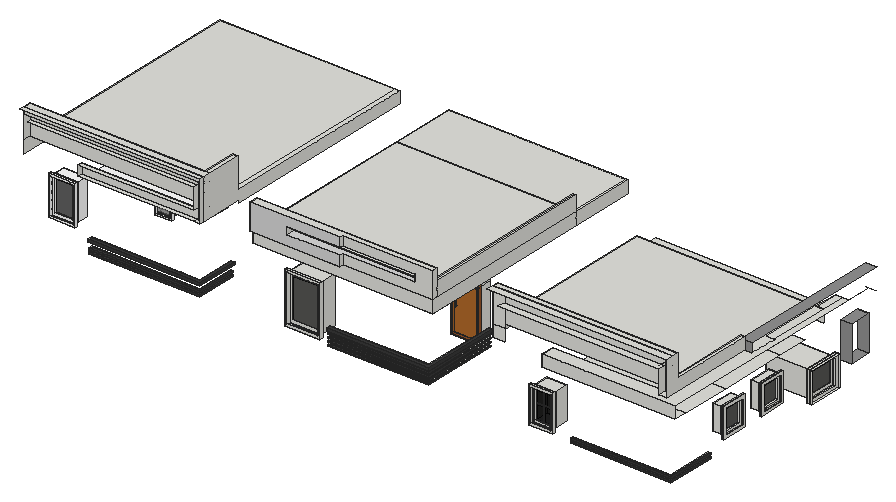
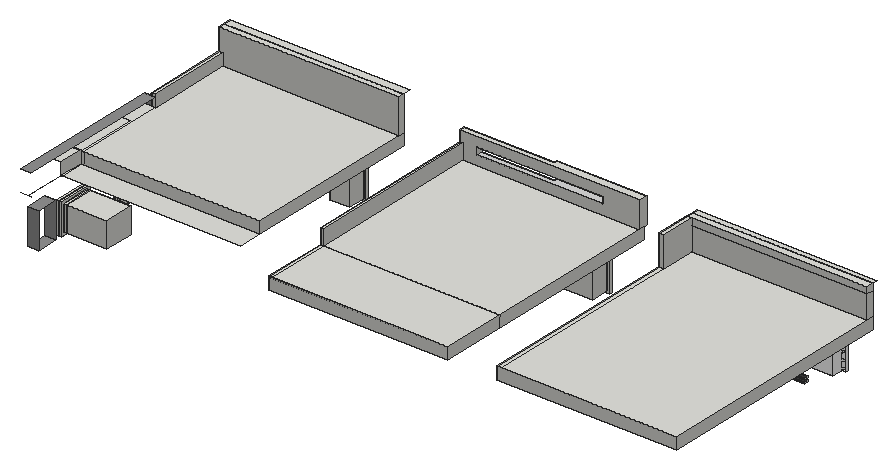
# SketchUp Ruby script. Lengths in inches.
U = 1.inch
M = Sketchup.active_model
def pt(a) = Geom::Point3d.new(a.map { |v| v * U })
def face(e, loops, mat)
  f = e.add_face(loops[0].map { |a| pt(a) })
  loops[1..].each { |l| e.add_face(l.map { |a| pt(a) }).erase! }
  f.material = f.back_material = mat if mat
  f
end
# faces: each face lists its corners as indices into pts; further lists are holes
def faces(e, pts, list, mat = nil) = list.each { |f| face(e, (f[0].is_a?(Array) ? f : [f]).map { |l| l.map { |i| pts[i] } }, mat) }
# xy, xz, yz: faces in a plane at the given z, y or x. An outline is a flat list of corners, or four numbers for a rectangle; further outlines are holes
def ring(l) = l.size == 4 ? [[l[0], l[1]], [l[2], l[1]], [l[2], l[3]], [l[0], l[3]]] : l.each_slice(2).to_a
def flat(e, list, mat, &to3) = list.each { |f| face(e, (f[0].is_a?(Array) ? f : [f]).map { |l| ring(l).map { |u, v| to3.(u, v) } }, mat) }
def xy(e, z, list, mat = nil) = flat(e, list, mat) { |x, y| [x, y, z] }
def xz(e, y, list, mat = nil) = flat(e, list, mat) { |x, z| [x, y, z] }
def yz(e, x, list, mat = nil) = flat(e, list, mat) { |y, z| [x, y, z] }
def lines(e, pts, list) = list.each { |a, b| e.add_line(pt(pts[a]), pt(pts[b])) }
# prism: a flat outline (further loops are holes) pulled along v
def prism(e, loops, v, mat = nil)
  f = face(e, loops, mat); d = Geom::Vector3d.new(v.map { |x| x * U })
  f.pushpull(f.normal.samedirection?(d) ? d.length : -d.length)
end
def box(e, o, s, mat = nil) = prism(e, [[o, [o[0] + s[0], o[1], o[2]], [o[0] + s[0], o[1] + s[1], o[2]], [o[0], o[1] + s[1], o[2]]]], [0, 0, s[2]], mat)
def at(x, y, z, deg = 0) = Geom::Transformation.translation(pt([x, y, z])) * Geom::Transformation.rotation(ORIGIN, Z_AXIS, deg.degrees)
def axes(o, x, y, z) = Geom::Transformation.new([*x, 0, *y, 0, *z, 0, *pt(o).to_a, 1])
def part(name) = M.definitions.add(name)
# library, detail: a bought-in or finely detailed component or shape, given as its bounding box
def library(name, o, s) = part(name).tap { |d| box(d.entities, o, s) }
def detail(e, o, s) = box(e.add_group.entities, o, s)
def put(e, d, t, mat = nil) = e.add_instance(d, t).tap { |i| i.material = mat if mat }
def group(e, t, mat = nil) = e.add_group.tap { |g| g.transformation = t; g.material = mat if mat }.entities
root = M.entities
M.materials.add("Generic").color = [145, 145, 145]
M.materials.add("Generic\#3").color = [216, 216, 216]
M.materials.add("[Color M00]").color = [255, 255, 255]
M.materials.add("[Color M07]").color = [58, 58, 58]
M.materials.add("[Color M08]").color = [45, 45, 45]
M.materials.add("[Translucent Glass Dark Green]").color = [168, 100, 12]
M.materials["[Translucent Glass Dark Green]"].alpha = 0.5
M.materials.add("[Translucent Glass Gray]").color = [0, 0, 0]
M.materials["[Translucent Glass Gray]"].alpha = 0.62
M.materials.add("[Translucent Glass Gray]1").color = [128, 128, 128]
M.materials["[Translucent Glass Gray]1"].alpha = 0.5
M.materials.add("[Wood Bamboo]").color = [177, 105, 43]
M.materials.add("[Wood Cherry Original]").color = [152, 86, 42]
c1 = part("Group\#10")
xy(c1.entities,0,[[0,1.08,55.8125,6.01]],"[Wood Cherry Original]")
xy(c1.entities,3.96,[[3.96,1.08,51.86,3.01]],"[Wood Bamboo]")
xy(c1.entities,51.66,[[8.63,0,9.88,3.01]],"[Color M08]")
xy(c1.entities,52.54,[[8.63,0.6875,9.88,3.01]],"[Color M08]")
xy(c1.entities,71.82,[[8.63,0.6875,9.88,3.01]],"[Color M08]")
xy(c1.entities,72.69,[[8.63,0,9.88,3.01]],"[Color M08]")
xy(c1.entities,97.36,[[3.96,1.08,51.86,3.01]],"[Wood Bamboo]")
xy(c1.entities,101.3125,[[0,1.08,55.8125,6.01]],"[Wood Bamboo]")
xy(c1.entities,102.55,[[1.23,1.08,27.29,3.01],[27.29,1.08,28.52,1.95],[28.52,1.08,54.58,3.01]],"[Wood Bamboo]")
xy(c1.entities,112.31,[[1.23,1.08,1.23,3.01,27.29,3.01,27.29,1.95,28.52,1.95,28.52,3.01,54.58,3.01,54.58,1.08]],"[Wood Bamboo]")
xy(c1.entities,113.54,[[0,1.08,55.8125,6.01]],"[Wood Bamboo]")
xz(c1.entities,0,[[8.63,51.66,9.88,72.69]],"[Color M08]")
xz(c1.entities,0.6875,[[8.63,52.54,9.88,71.82]])
xz(c1.entities,1.08,[[0,101.3125,55.8125,102.55],[0,102.55,1.23,102.55,1.23,112.31,54.58,112.31,54.58,102.55,55.8125,102.55,55.8125,113.54,0,113.54]],"[Wood Bamboo]")
xz(c1.entities,1.08,[[[0,0,55.8125,101.3125],[3.96,3.96,51.86,97.36]]],"[Wood Cherry Original]")
xz(c1.entities,1.95,[[27.29,102.55,28.52,112.31]],"[Wood Bamboo]")
xz(c1.entities,3.01,[[8.63,71.82,9.88,72.69]])
xz(c1.entities,3.01,[[1.23,102.55,27.29,112.31],[28.52,102.55,54.58,112.31]],"[Translucent Glass Dark Green]")
xz(c1.entities,3.01,[[[3.96,3.96,51.86,97.36],[8.63,71.82,9.88,72.69],[8.63,51.66,9.88,52.54]]],"[Wood Bamboo]")
xz(c1.entities,6.01,[[0,0,55.8125,101.3125],[0,112.31,55.8125,113.54]],"[Wood Bamboo]")
yz(c1.entities,0,[[1.08,101.3125,6.01,113.54]],"[Wood Bamboo]")
yz(c1.entities,0,[[1.08,0,6.01,101.3125]],"[Wood Cherry Original]")
yz(c1.entities,1.23,[[1.08,102.55,3.01,112.31]],"[Wood Bamboo]")
yz(c1.entities,3.96,[[1.08,3.96,3.01,97.36]],"[Wood Bamboo]")
yz(c1.entities,8.63,[[0,51.66,0,72.69,3.01,72.69,3.01,71.82,0.6875,71.82,0.6875,52.54,3.01,52.54,3.01,51.66]],"[Color M08]")
yz(c1.entities,9.88,[[0,51.66,3.01,51.66,3.01,52.54,0.6875,52.54,0.6875,71.82,3.01,71.82,3.01,72.69,0,72.69]],"[Color M08]")
yz(c1.entities,27.29,[[1.95,102.55,3.01,112.31]],"[Wood Bamboo]")
yz(c1.entities,28.52,[[1.95,102.55,3.01,112.31]],"[Wood Bamboo]")
yz(c1.entities,51.86,[[1.08,3.96,3.01,97.36]],"[Wood Bamboo]")
yz(c1.entities,54.58,[[1.08,102.55,3.01,112.31]],"[Wood Bamboo]")
yz(c1.entities,55.8125,[[1.08,101.3125,6.01,113.54]],"[Wood Bamboo]")
yz(c1.entities,55.8125,[[1.08,0,6.01,101.3125]],"[Wood Cherry Original]")
p = [[1.23,3.01,112.31],[1.23,6.01,112.31],[9.24,3.01,71.99],[9.24,0.51,71.99],[9.24,0.51,52.37],[9.24,3.01,52.37]]
lines(c1.entities,p,[[0,1],[2,3],[3,4],[4,5]])
c2 = part("Group\#1")
xy(c2.entities,0,[[0,0,39.9375,6]])
xy(c2.entities,3.79,[[3.79,0,36.15,3]])
xy(c2.entities,60.83,[[3.79,0,36.15,3]])
xy(c2.entities,64.62,[[0,0,39.9375,6]])
xz(c2.entities,0,[[[0,0,39.9375,64.62],[3.79,3.79,36.15,60.83]]])
xz(c2.entities,3,[[18.07,3.79,20.49,3.79,20.49,32.1,36.15,32.1,36.15,34.21,20.49,34.21,20.49,60.83,18.07,60.83,18.07,34.21,3.79,34.21,3.79,32.1,18.07,32.1]],"[Color M08]")
xz(c2.entities,3,[[3.79,3.79,18.07,32.1],[20.49,3.79,36.15,32.1],[3.79,34.21,18.07,60.83],[20.49,34.21,36.15,60.83]],"[Translucent Glass Gray]")
xz(c2.entities,6,[[0,0,39.9375,64.62]],"[Translucent Glass Gray]")
yz(c2.entities,0,[[0,0,6,64.62]])
yz(c2.entities,3.79,[[0,3.79,3,60.83]])
yz(c2.entities,36.15,[[0,3.79,3,60.83]])
yz(c2.entities,39.9375,[[0,0,6,64.62]])
c3 = part("Group\#8")
xy(c3.entities,0,[[0,0,6,59.4375]])
xy(c3.entities,4.64,[[3,4.64,6,54.8]])
xy(c3.entities,46.99,[[3,4.64,6,54.8]])
xy(c3.entities,51.625,[[0,0,6,59.4375]])
xz(c3.entities,0,[[0,0,6,51.625]])
xz(c3.entities,4.64,[[3,4.64,6,46.99]])
xz(c3.entities,54.8,[[3,4.64,6,46.99]])
xz(c3.entities,59.4375,[[0,0,6,51.625]])
yz(c3.entities,0,[[0,0,59.4375,51.625]])
yz(c3.entities,3,[[4.64,4.64,54.8,46.99]],"[Translucent Glass Gray]")
yz(c3.entities,6,[[[0,0,59.4375,51.625],[4.64,4.64,54.8,46.99]]])
c4 = part("Group\#2")
xy(c4.entities,0,[[0,0,62.4375,3]])
xy(c4.entities,93.0625,[[0,0,62.4375,3]])
xz(c4.entities,0,[[[0,0,62.4375,93.0625],[6.31,6.31,56.13,86.75]]])
xz(c4.entities,0,[[6.31,6.31,56.13,86.75]],"[Translucent Glass Gray]")
xz(c4.entities,3,[[0,0,62.4375,93.0625]])
yz(c4.entities,0,[[0,0,3,93.0625]])
yz(c4.entities,62.4375,[[0,0,3,93.0625]])
c5 = part("Group\#6")
xy(c5.entities,0,[[0,0,6,44.5]])
xy(c5.entities,4.57,[[3,4.57,6,39.93]])
xy(c5.entities,45.43,[[3,4.57,6,39.93]])
xy(c5.entities,50,[[0,0,6,44.5]])
xz(c5.entities,0,[[0,0,6,50]])
xz(c5.entities,4.57,[[3,4.57,6,45.43]])
xz(c5.entities,39.93,[[3,4.57,6,45.43]])
xz(c5.entities,44.5,[[0,0,6,50]])
yz(c5.entities,0,[[0,0,44.5,50]])
yz(c5.entities,3,[[4.57,4.57,39.93,45.43]],"[Translucent Glass Gray]")
yz(c5.entities,6,[[[0,0,44.5,50],[4.57,4.57,39.93,45.43]]])
c6 = part("Group\#5")
xy(c6.entities,0,[[0,0,46.6875,6]],"[Color M00]")
xy(c6.entities,4.48,[[4.48,0,42.2,3]],"[Color M00]")
xy(c6.entities,67.45,[[4.48,0,42.2,3]],"[Color M00]")
xy(c6.entities,71.9375,[[0,0,46.6875,6]],"[Color M00]")
xz(c6.entities,0,[[[0,0,46.6875,71.9375],[4.48,4.48,42.2,67.45]]],"[Color M00]")
xz(c6.entities,3,[[4.48,4.48,42.2,67.45]],"[Translucent Glass Gray]")
xz(c6.entities,6,[[0,0,46.6875,71.9375]],"[Color M00]")
yz(c6.entities,0,[[0,0,6,71.9375]],"[Color M00]")
yz(c6.entities,4.48,[[0,4.48,3,67.45]],"[Color M00]")
yz(c6.entities,42.2,[[0,4.48,3,67.45]],"[Color M00]")
yz(c6.entities,46.6875,[[0,0,6,71.9375]],"[Color M00]")
c7 = part("Group\#11")
xy(c7.entities,0,[[0,0,27.8125,3]])
xy(c7.entities,27.8125,[[0,0,27.8125,3]])
xz(c7.entities,0,[[0,0,27.8125,27.8125]],"[Translucent Glass Gray]1")
xz(c7.entities,3,[[0,0,27.8125,27.8125]],"[Translucent Glass Gray]1")
yz(c7.entities,0,[[0,0,3,27.8125]])
yz(c7.entities,27.8125,[[0,0,3,27.8125]])
c8 = part("Group\#12")
xy(c8.entities,0,[[0,0,20.25,3]])
xy(c8.entities,24.8125,[[0,0,20.25,3]])
xz(c8.entities,0,[[0,0,20.25,24.8125]],"[Translucent Glass Gray]1")
xz(c8.entities,3,[[0,0,20.25,24.8125]],"[Translucent Glass Gray]1")
yz(c8.entities,0,[[0,0,3,24.8125]])
yz(c8.entities,20.25,[[0,0,3,24.8125]])
xy(root,990.21,[[863.52,258.8125,919.33,288.3125]])
xy(root,991.25,[[263.03,103.78,263.03,109.42,479.41,109.42,479.41,187.125,485.0625,187.125,485.0625,103.78]],"[Color M07]")
xy(root,991.4375,[[1230.96,101.06,1230.96,106.62,1426.46,106.62,1426.46,199.25,1432.02,199.25,1432.02,101.06]],"[Color M07]")
xy(root,994.1875,[[1230.96,101.06,1432.02,101.06,1432.02,199.25,1426.46,199.25,1426.46,106.62,1230.96,106.62]],"[Color M07]")
xy(root,994.52,[[741.96,102.9375,741.96,107.75,939.83,107.75,939.83,258.8125,944.64,258.8125,944.64,102.9375]],"[Color M07]")
xy(root,994.62,[[263.03,103.78,485.0625,103.78,485.0625,187.125,479.41,187.125,479.41,109.42,263.03,109.42]],"[Color M07]")
xy(root,996.39,[[741.96,102.9375,944.64,102.9375,944.64,258.8125,939.83,258.8125,939.83,107.75,741.96,107.75]],"[Color M07]")
xy(root,998.31,[[263.03,103.78,263.03,109.42,479.41,109.42,479.41,187.125,485.0625,187.125,485.0625,103.78]],"[Color M07]")
xy(root,998.375,[[1230.96,101.06,1230.96,106.62,1426.46,106.62,1426.46,199.25,1432.02,199.25,1432.02,101.06]],"[Color M07]")
xy(root,1000.39,[[1151.9,93.8125,1200.57,99.8125]])
xy(root,1001.125,[[1230.96,101.06,1432.02,101.06,1432.02,199.25,1426.46,199.25,1426.46,106.62,1230.96,106.62]],"[Color M07]")
xy(root,1001.68,[[263.03,103.78,485.0625,103.78,485.0625,187.125,479.41,187.125,479.41,109.42,263.03,109.42]],"[Color M07]")
xy(root,1001.7,[[741.96,102.9375,741.96,107.75,939.83,107.75,939.83,258.8125,944.64,258.8125,944.64,102.9375]],"[Color M07]")
xy(root,1002.85,[[1452.58,416.24,1457.58,486.33],[1457.58,416.24,1462.21,486.33]])
xy(root,1003.57,[[741.96,102.9375,944.64,102.9375,944.64,258.8125,939.83,258.8125,939.83,107.75,741.96,107.75]],"[Color M07]")
xy(root,1004.75,[[1156.27,93.8125,1196.2,99.8125],[1156.27,99.8125,1196.2,134.3125]])
xy(root,1006.65,[[663.18,93.8125,734.35,99.8125]])
xy(root,1008.18,[[1365.64,421.57,1452.58,481],[1452.58,421.57,1457.58,481]])
xy(root,1008.5625,[[741.96,102.9375,741.96,107.75,939.83,107.75,939.83,258.8125,944.64,258.8125,944.64,102.9375]],"[Color M07]")
xy(root,1010.4375,[[741.96,102.9375,944.64,102.9375,944.64,258.8125,939.83,258.8125,939.83,107.75,741.96,107.75]],"[Color M07]")
xy(root,1011.02,[[667.55,93.8125,729.98,99.8125],[667.55,99.8125,729.98,136.8125]])
xy(root,1013.31,[[263.03,101.4,263.03,109.42,479.41,109.42,479.41,187.125,487.4375,187.125,487.4375,101.4]],"[Color M07]")
xy(root,1015.6875,[[741.96,102.9375,741.96,107.75,939.83,107.75,939.83,258.8125,944.64,258.8125,944.64,102.9375]],"[Color M07]")
xy(root,1017.5625,[[741.96,102.9375,944.64,102.9375,944.64,258.8125,939.83,258.8125,939.83,107.75,741.96,107.75]],"[Color M07]")
xy(root,1017.77,[[1435.83,223.32,1439.83,276.63],[1435.83,318.51,1439.83,371.82]])
xy(root,1017.95,[[303.36,105.3,304.92,108.8],[306.11,105.3,307.67,108.8],[441.9,105.3,443.46,109.43],[444.65,105.3,446.21,109.43]])
xy(root,1018.25,[[263.03,101.4,487.4375,101.4,487.4375,187.125,479.41,187.125,479.41,109.42,263.03,109.42]],"[Color M07]")
xy(root,1022.17,[[1414.21,227.73,1435.83,272.23],[1435.83,227.73,1439.83,272.23],[1414.21,322.92,1435.83,367.42],[1435.83,322.92,1439.83,367.42]])
xy(root,1022.6875,[[741.96,99.8125,741.96,107.75,939.83,107.75,939.83,258.8125,947.77,258.8125,947.77,99.8125]],"[Color M07]")
xy(root,1023.75,[[1429.21,528.77,1451.02,572.96]],"Generic")
xy(root,1028.125,[[741.96,99.8125,947.77,99.8125,947.77,258.8125,939.83,258.8125,939.83,107.75,741.96,107.75]],"[Color M07]")
xy(root,1034.32,[[188.42,94.8125,242.3125,99.8125]],"[Color M00]")
xy(root,1037.92,[[192.03,94.8125,238.71,128.125]],"[Color M00]")
xy(root,1051,[[331.98,182.0625,365.3125,187.125]],"[Color M00]")
xy(root,1053.76,[[334.74,187.125,362.55,221.125]])
xy(root,1053.76,[[334.74,182.0625,362.55,187.125]],"[Color M00]")
xy(root,1055.54,[[1292.01,194.1875,1317.77,199.25]])
xy(root,1058.29,[[1294.76,194.1875,1315.01,199.25],[1294.76,199.25,1315.01,212.4375]])
xy(root,1059.8,[[1365.64,421.57,1452.58,481],[1452.58,421.57,1457.58,481]])
xy(root,1065.125,[[1452.58,416.24,1457.58,486.33],[1457.58,416.24,1462.21,486.33]])
xy(root,1069.375,[[1156.27,93.8125,1196.2,99.8125],[1156.27,99.8125,1196.2,134.3125]])
xy(root,1069.84,[[808.05,253.75,841.375,258.8125]])
xy(root,1072.17,[[1414.21,227.73,1435.83,272.23],[1435.83,227.73,1439.83,272.23],[1414.21,322.92,1435.83,367.42],[1435.83,322.92,1439.83,367.42]])
xy(root,1072.6,[[810.81,253.75,838.62,258.8125],[810.81,258.8125,838.62,292.8125]])
xy(root,1073.74,[[1151.9,93.8125,1200.57,99.8125]])
xy(root,1076.58,[[1435.83,223.32,1439.83,276.63],[1435.83,318.51,1439.83,371.82]])
xy(root,1081.57,[[334.74,187.125,362.55,221.125]])
xy(root,1081.57,[[334.74,182.0625,362.55,187.125]],"[Color M00]")
xy(root,1083.11,[[1294.76,194.1875,1315.01,199.25],[1294.76,199.25,1315.01,212.4375]])
xy(root,1084.33,[[331.98,182.0625,365.3125,187.125]],"[Color M00]")
xy(root,1085.86,[[1292.01,194.1875,1317.77,199.25]])
xy(root,1088.1,[[1327.46,199.25,1383.27,240]])
xy(root,1095.24,[[1429.21,528.77,1451.02,572.96]],"Generic")
xy(root,1100.41,[[810.81,253.75,838.62,258.8125],[810.81,258.8125,838.62,292.8125]])
xy(root,1101.01,[[391.33,187.125,447.14,220.9375]],"[Color M00]")
xy(root,1103.17,[[808.05,253.75,841.375,258.8125]])
xy(root,1104.02,[[863.52,258.8125,919.33,288.3125]])
xy(root,1104.08,[[667.55,93.8125,729.98,99.8125],[667.55,99.8125,729.98,136.8125]])
xy(root,1108.45,[[663.18,93.8125,734.35,99.8125]])
xy(root,1109.85,[[192.03,94.8125,238.71,128.125]],"[Color M00]")
xy(root,1113.45,[[188.42,94.8125,242.3125,99.8125]],"[Color M00]")
xy(root,1128,[[1195.78,73.25,1230.96,99.8125],[1230.96,73.25,1462.21,99.8125],[594.11,99.8125,594.11,459.8125,954.11,459.8125,954.11,258.8125,741.96,258.8125,741.96,99.8125],[741.96,99.8125,954.11,258.8125],[1230.96,99.8125,1462.21,199.25],
  [1435.83,199.25,1462.21,336.18],[1433.58,336.18,1435.83,398.12],[1435.83,336.18,1462.21,398.12],[594.11,459.8125,954.11,590.625],[1075.83,459.8125,1433.58,507.5625],
  [1433.58,459.8125,1435.83,507.5625],[1433.58,507.5625,1435.83,507.75]])
xy(root,1132.1875,[[250.57,90.625,483.3125,99.8125],[483.3125,90.625,495.5,99.8125]])
xy(root,1132.1875,[[263.03,99.8125,495.5,187.125]],"[Color M00]")
xy(root,1152,[[1195.78,73.25,1462.21,73.25,1462.21,507.75,1451.02,507.75,1451.02,279.74,1435.83,279.74,1435.83,84.125,1420.08,84.125,1420.08,99.8125,1195.78,99.8125],[1420.08,84.125,1435.83,99.8125],[250.57,90.625,483.3125,99.8125],[594.11,93.3125,773.96,99.8125],[594.11,99.8125,954.11,111.1875],
  [594.11,111.1875,948.42,459.8125],[948.42,111.1875,954.11,459.8125],[1075.83,111.625,1429.21,459.8125],[1429.21,111.625,1435.83,279.74],[135.5,114.875,486.0625,590.625],
  [486.0625,185.16,495.5,590.625],[1429.21,279.74,1429.21,459.8125,1433.58,459.8125,1433.58,336.18,1451.02,336.18,1451.02,279.74],[1433.58,336.18,1451.02,459.8125],[594.11,459.8125,948.42,590.625],[948.42,459.8125,954.11,590.625],
  [1435.83,459.8125,1451.02,507.75]])
xy(root,1170.6875,[[1429.21,279.74,1451.02,591.3125]],"Generic")
xy(root,1172.34,[[668.04,93.3125,773.96,93.3125,773.96,99.8125,919.97,99.8125,919.97,111.1875,668.04,111.1875]],"Generic\#3")
xy(root,1176.75,[[1429.21,111.625,1435.83,279.74]])
xy(root,1182.4375,[[948.42,111.1875,954.11,459.8125]])
xy(root,1186.66,[[668.04,93.3125,668.04,111.1875,919.97,111.1875,919.97,99.8125,773.96,99.8125,773.96,93.3125]])
xy(root,1193.875,[[150.0625,90.625,483.3125,99.8125]])
xy(root,1198.4375,[[1098.52,84.125,1420.08,99.8125]])
xy(root,1204.625,[[594.11,93.3125,773.96,93.3125,773.96,99.8125,954.11,99.8125,954.11,111.1875,594.11,111.1875]])
xy(root,1212.3125,[[135.5,90.625,495.5,99.8125],[135.5,99.8125,495.5,114.875],[486.0625,114.875,495.5,185.16]])
xy(root,1221,[[1075.83,84.125,1435.83,99.8125],[1075.83,99.8125,1435.83,111.625]])
xz(root,73.25,[[1195.78,1128,1462.21,1152]])
xz(root,93.3125,[[594.11,1152,773.96,1152,773.96,1172.34,668.04,1172.34,668.04,1186.66,773.96,1186.66,773.96,1204.625,594.11,1204.625]],"Generic\#3")
xz(root,93.8125,[[[1151.9,1000.39,1200.57,1073.74],[1156.27,1004.75,1196.2,1069.375]],[[663.18,1006.65,734.35,1108.45],[667.55,1011.02,729.98,1104.08]]])
xz(root,94.8125,[[[188.42,1034.32,242.3125,1113.45],[192.03,1037.92,238.71,1109.85]]],"[Color M00]")
xz(root,99.8125,[[[1151.9,1000.39,1200.57,1073.74],[1156.27,1004.75,1196.2,1069.375]],[[663.18,1006.65,734.35,1108.45],[667.55,1011.02,729.98,1104.08]],[594.11,1128,954.11,1152],[1075.83,1128,1098.52,1152],[250.57,1132.1875,483.3125,1152],
  [483.3125,1132.1875,495.5,1152],[483.3125,1152,495.5,1198.3125],[773.96,1152,954.11,1152,954.11,1204.625,773.96,1204.625,773.96,1186.66,919.97,1186.66,919.97,1172.34,773.96,1172.34],[1075.83,1152,1098.52,1221],[150.0625,1193.875,483.3125,1198.3125],
  [135.5,1198.3125,495.5,1212.3125],[1098.52,1198.4375,1420.08,1221]])
xz(root,99.8125,[[741.96,1022.6875,947.77,1028.125]],"[Color M07]")
xz(root,101.06,[[1230.96,991.4375,1432.02,994.1875],[1230.96,998.375,1432.02,1001.125]],"[Color M07]")
xz(root,101.4,[[263.03,1013.31,487.4375,1018.25]],"[Color M07]")
xz(root,102.9375,[[741.96,994.52,944.64,996.39],[741.96,1001.7,944.64,1003.57],[741.96,1008.5625,944.64,1010.4375],[741.96,1015.6875,944.64,1017.5625]],"[Color M07]")
xz(root,103.78,[[263.03,991.25,485.0625,994.62],[263.03,998.31,485.0625,1001.68]],"[Color M07]")
xz(root,106.62,[[1230.96,991.4375,1426.46,994.1875],[1230.96,998.375,1426.46,1001.125]])
xz(root,107.75,[[741.96,994.52,939.83,996.39],[741.96,1001.7,939.83,1003.57],[741.96,1008.5625,939.83,1010.4375],[741.96,1015.6875,939.83,1017.5625],[741.96,1022.6875,939.83,1028.125]])
xz(root,109.42,[[263.03,991.25,479.41,994.62],[263.03,998.31,479.41,1001.68],[263.03,1013.31,479.41,1018.25]])
xz(root,111.1875,[[[594.11,1152,594.11,1204.625,954.11,1204.625,954.11,1182.4375,948.42,1182.4375,948.42,1152],[668.04,1172.34,919.97,1186.66]],[948.42,1152,954.11,1182.4375]])
xz(root,111.625,[[1075.83,1152,1075.83,1221,1435.83,1221,1435.83,1176.75,1429.21,1176.75,1429.21,1152]])
xz(root,114.875,[[135.5,1152,486.0625,1198.3125],[135.5,1198.3125,486.0625,1212.3125]])
xz(root,128.125,[[192.03,1037.92,238.71,1109.85]],"[Color M00]")
xz(root,134.3125,[[1156.27,1004.75,1196.2,1069.375]])
xz(root,136.8125,[[667.55,1011.02,729.98,1104.08]])
xz(root,182.0625,[[[331.98,1051,365.3125,1084.33],[334.74,1053.76,362.55,1081.57]]],"[Color M00]")
xz(root,185.16,[[486.0625,1152,495.5,1212.3125]])
xz(root,187.125,[[[331.98,1051,365.3125,1084.33],[334.74,1053.76,362.55,1081.57]]],"[Color M00]")
xz(root,194.1875,[[[1292.01,1055.54,1317.77,1085.86],[1294.76,1058.29,1315.01,1083.11]]])
xz(root,199.25,[[[1292.01,1055.54,1317.77,1085.86],[1294.76,1058.29,1315.01,1083.11]]])
xz(root,212.4375,[[1294.76,1058.29,1315.01,1083.11]])
xz(root,220.9375,[[391.33,1087.12,447.14,1101.01]],"[Color M00]")
xz(root,221.125,[[334.74,1053.76,362.55,1081.57]])
xz(root,223.32,[[1435.83,1017.77,1439.83,1076.58]])
xz(root,227.73,[[1414.21,1022.17,1435.83,1072.17],[1435.83,1022.17,1439.83,1072.17]])
xz(root,240,[[1327.46,1075.87,1383.27,1088.1]])
xz(root,253.75,[[[808.05,1069.84,841.375,1103.17],[810.81,1072.6,838.62,1100.41]]])
xz(root,258.8125,[[[808.05,1069.84,841.375,1103.17],[810.81,1072.6,838.62,1100.41]]])
xz(root,272.23,[[1414.21,1022.17,1435.83,1072.17],[1435.83,1022.17,1439.83,1072.17]])
xz(root,276.63,[[1435.83,1017.77,1439.83,1076.58]])
xz(root,279.74,[[1429.21,1152,1435.83,1170.6875],[1429.21,1170.6875,1435.83,1176.75]])
xz(root,279.74,[[1435.83,1152,1451.02,1170.6875]],"Generic")
xz(root,288.3125,[[863.52,990.21,919.33,1091.52],[863.52,1091.52,919.33,1104.02]])
xz(root,292.8125,[[810.81,1072.6,838.62,1100.41]])
xz(root,318.51,[[1435.83,1017.77,1439.83,1076.58]])
xz(root,322.92,[[1414.21,1022.17,1435.83,1072.17],[1435.83,1022.17,1439.83,1072.17]])
xz(root,367.42,[[1414.21,1022.17,1435.83,1072.17],[1435.83,1022.17,1439.83,1072.17]])
xz(root,371.82,[[1435.83,1017.77,1439.83,1076.58]])
xz(root,416.24,[[1452.58,1002.85,1457.58,1065.125],[1457.58,1002.85,1462.21,1065.125]])
xz(root,421.57,[[1365.64,1008.18,1452.58,1059.8],[1452.58,1008.18,1457.58,1059.8]])
xz(root,459.8125,[[594.11,1128,954.11,1152],[1075.83,1128,1429.21,1152],[1429.21,1128,1433.58,1152],[1433.58,1128,1435.83,1152],[1435.83,1128,1451.02,1152],
  [948.42,1152,954.11,1182.4375]])
xz(root,481,[[1365.64,1008.18,1452.58,1059.8],[1452.58,1008.18,1457.58,1059.8]])
xz(root,486.33,[[1452.58,1002.85,1457.58,1065.125],[1457.58,1002.85,1462.21,1065.125]])
xz(root,528.77,[[1429.21,1023.75,1451.02,1095.24]],"Generic")
xz(root,572.96,[[1429.21,1023.75,1451.02,1095.24]],"Generic")
xz(root,590.625,[[135.5,1128,495.5,1152],[594.11,1128,954.11,1152]])
yz(root,135.5,[[99.8125,1128,590.625,1152],[99.8125,1152,114.875,1198.3125],[99.8125,1198.3125,114.875,1212.3125]])
yz(root,188.42,[[94.8125,1034.32,99.8125,1113.45]],"[Color M00]")
yz(root,192.03,[[94.8125,1037.92,128.125,1109.85]],"[Color M00]")
yz(root,238.71,[[94.8125,1037.92,128.125,1109.85]],"[Color M00]")
yz(root,242.3125,[[94.8125,1034.32,99.8125,1113.45]],"[Color M00]")
yz(root,250.57,[[90.625,1132.1875,99.8125,1152]])
yz(root,263.03,[[103.78,991.25,109.42,994.62],[103.78,998.31,109.42,1001.68],[101.4,1013.31,109.42,1018.25]])
yz(root,331.98,[[182.0625,1051,187.125,1084.33]],"[Color M00]")
yz(root,334.74,[[187.125,1053.76,221.125,1081.57]])
yz(root,334.74,[[182.0625,1053.76,187.125,1081.57]],"[Color M00]")
yz(root,362.55,[[187.125,1053.76,221.125,1081.57]])
yz(root,362.55,[[182.0625,1053.76,187.125,1081.57]],"[Color M00]")
yz(root,365.3125,[[182.0625,1051,187.125,1084.33]],"[Color M00]")
yz(root,391.33,[[187.125,1087.12,220.9375,1101.01]],"[Color M00]")
yz(root,447.14,[[187.125,1087.12,220.9375,1101.01]],"[Color M00]")
yz(root,479.41,[[109.42,991.25,187.125,994.62],[109.42,998.31,187.125,1001.68],[109.42,1013.31,187.125,1018.25]])
yz(root,483.3125,[[90.625,1152,99.8125,1193.875]])
yz(root,485.0625,[[103.78,991.25,187.125,994.62],[103.78,998.31,187.125,1001.68]],"[Color M07]")
yz(root,486.0625,[[114.875,1152,185.16,1212.3125]])
yz(root,487.4375,[[101.4,1013.31,187.125,1018.25]],"[Color M07]")
yz(root,495.5,[[187.125,1128,590.625,1128,590.625,1152,185.16,1152,185.16,1212.3125,99.8125,1212.3125,99.8125,1132.1875,187.125,1132.1875],[90.625,1132.1875,99.8125,1212.3125]])
yz(root,594.11,[[99.8125,1128,459.8125,1152],[459.8125,1128,590.625,1152],[93.3125,1152,111.1875,1204.625]])
yz(root,663.18,[[93.8125,1006.65,99.8125,1108.45]])
yz(root,667.55,[[93.8125,1011.02,99.8125,1104.08],[99.8125,1011.02,136.8125,1104.08]])
yz(root,668.04,[[93.3125,1172.34,111.1875,1186.66]])
yz(root,729.98,[[93.8125,1011.02,99.8125,1104.08],[99.8125,1011.02,136.8125,1104.08]])
yz(root,734.35,[[93.8125,1006.65,99.8125,1108.45]])
yz(root,741.96,[[102.9375,994.52,107.75,996.39],[102.9375,1001.7,107.75,1003.57],[102.9375,1008.5625,107.75,1010.4375],[102.9375,1015.6875,107.75,1017.5625],[99.8125,1022.6875,107.75,1028.125]])
yz(root,773.96,[[93.3125,1152,99.8125,1172.34],[93.3125,1186.66,99.8125,1204.625]])
yz(root,808.05,[[253.75,1069.84,258.8125,1103.17]])
yz(root,810.81,[[253.75,1072.6,258.8125,1100.41],[258.8125,1072.6,292.8125,1100.41]])
yz(root,838.62,[[253.75,1072.6,258.8125,1100.41],[258.8125,1072.6,292.8125,1100.41]])
yz(root,841.375,[[253.75,1069.84,258.8125,1103.17]])
yz(root,863.52,[[258.8125,990.21,288.3125,1091.52],[258.8125,1091.52,288.3125,1104.02]])
yz(root,919.33,[[258.8125,990.21,288.3125,1091.52],[258.8125,1091.52,288.3125,1104.02]])
yz(root,919.97,[[99.8125,1172.34,111.1875,1186.66]])
yz(root,939.83,[[107.75,994.52,258.8125,996.39],[107.75,1001.7,258.8125,1003.57],[107.75,1008.5625,258.8125,1010.4375],[107.75,1015.6875,258.8125,1017.5625],[107.75,1022.6875,258.8125,1028.125]])
yz(root,944.64,[[102.9375,994.52,258.8125,996.39],[102.9375,1001.7,258.8125,1003.57],[102.9375,1008.5625,258.8125,1010.4375],[102.9375,1015.6875,258.8125,1017.5625]],"[Color M07]")
yz(root,947.77,[[99.8125,1022.6875,258.8125,1028.125]],"[Color M07]")
yz(root,948.42,[[111.1875,1152,459.8125,1182.4375]])
yz(root,954.11,[[99.8125,1128,459.8125,1152],[459.8125,1128,590.625,1152],[99.8125,1152,111.1875,1204.625],[111.1875,1152,459.8125,1182.4375]])
yz(root,1075.83,[[99.8125,1128,459.8125,1152],[99.8125,1152,111.625,1221]])
yz(root,1151.9,[[93.8125,1000.39,99.8125,1073.74]])
yz(root,1156.27,[[93.8125,1004.75,99.8125,1069.375],[99.8125,1004.75,134.3125,1069.375]])
yz(root,1195.78,[[73.25,1128,99.8125,1152]])
yz(root,1196.2,[[93.8125,1004.75,99.8125,1069.375],[99.8125,1004.75,134.3125,1069.375]])
yz(root,1200.57,[[93.8125,1000.39,99.8125,1073.74]])
yz(root,1230.96,[[101.06,991.4375,106.62,994.1875],[101.06,998.375,106.62,1001.125]])
yz(root,1292.01,[[194.1875,1055.54,199.25,1085.86]])
yz(root,1294.76,[[194.1875,1058.29,199.25,1083.11],[199.25,1058.29,212.4375,1083.11]])
yz(root,1315.01,[[194.1875,1058.29,199.25,1083.11],[199.25,1058.29,212.4375,1083.11]])
yz(root,1317.77,[[194.1875,1055.54,199.25,1085.86]])
yz(root,1327.46,[[199.25,1075.87,240,1088.1]])
yz(root,1365.64,[[421.57,1008.18,481,1059.8]])
yz(root,1383.27,[[199.25,1075.87,240,1088.1]])
yz(root,1414.21,[[227.73,1022.17,272.23,1072.17],[322.92,1022.17,367.42,1072.17]])
yz(root,1420.08,[[84.125,1152,99.8125,1198.4375]])
yz(root,1426.46,[[106.62,991.4375,199.25,994.1875],[106.62,998.375,199.25,1001.125]])
yz(root,1429.21,[[111.625,1152,279.74,1176.75]])
yz(root,1432.02,[[101.06,991.4375,199.25,994.1875],[101.06,998.375,199.25,1001.125]],"[Color M07]")
yz(root,1435.83,[[[223.32,1017.77,276.63,1076.58],[227.73,1022.17,272.23,1072.17]],[[318.51,1017.77,371.82,1076.58],[322.92,1022.17,367.42,1072.17]],[459.8125,1128,507.75,1152],[84.125,1152,279.74,1152,279.74,1176.75,111.625,1176.75,111.625,1221,84.125,1221]])
yz(root,1439.83,[[[223.32,1017.77,276.63,1076.58],[227.73,1022.17,272.23,1072.17]],[[318.51,1017.77,371.82,1076.58],[322.92,1022.17,367.42,1072.17]]])
yz(root,1452.58,[[[416.24,1002.85,486.33,1065.125],[421.57,1008.18,481,1059.8]]])
yz(root,1457.58,[[[416.24,1002.85,486.33,1065.125],[421.57,1008.18,481,1059.8]]])
p = [[486.0625,114.875,1152],[495.5,114.875,1152],[486.0625,114.875,1198.3125],[495.5,114.875,1198.3125],[263.03,105.8125,993],[483.03,105.8125,993],
  [483.03,187.125,993],[263.03,105.8125,1000],[483.03,105.8125,1000],[483.03,187.125,1000],[263.03,105.8125,1015],[483.03,105.8125,1015],
  [483.03,187.125,1015],[1420.08,99.8125,1204.6875],[1435.83,99.8125,1204.6875],[1420.08,84.125,1204.6875],[741.96,105.47,995.6875],[942.11,105.47,995.6875],
  [942.11,258.8125,995.6875],[942.11,105.47,1002.6875],[942.11,258.8125,1002.6875],[741.96,105.47,1002.6875],[942.11,105.47,1009.6875],[942.11,258.8125,1009.6875],
  [741.96,105.47,1009.6875],[942.11,105.47,1016.6875],[942.11,258.8125,1016.6875],[741.96,105.47,1016.6875],[942.11,105.47,1023.6875],[942.11,258.8125,1023.6875],
  [741.96,105.47,1023.6875],[1230.96,103.125,993],[1429.96,103.125,993],[1429.96,199.25,993],[1230.96,103.125,1000],[1429.96,103.125,1000],
  [1429.96,199.25,1000],[1435.83,507.75,1128],[1435.83,590.625,1128],[1429.21,590.625,1128],[1429.21,591.3125,1128],[1451.02,590.625,1128],
  [1451.02,591.3125,1128]]
lines(root,p,[[0,1],[2,3],[4,5],[5,6],[7,8],[8,9],[10,11],[11,12],[13,14],[13,15],[16,17],[17,18],
  [19,20],[21,19],[22,23],[24,22],[25,26],[27,25],[28,29],[30,28],[31,32],[32,33],[34,35],[35,36],
  [37,38],[39,40],[41,42],[39,38],[38,41]])
put(root,c1,at(863.52,258.8125,990.47))
put(root,c2,at(1156.45,99.8125,1004.75))
put(root,c3,at(1446.58,421.57,1008.18))
put(root,c4,at(667.55,99.8125,1011.02))
put(root,c5,at(1429.83,227.73,1022.17))
put(root,c5,at(1429.83,322.92,1022.17))
put(root,c6,at(192.03,99.8125,1037.92))
put(root,c7,at(334.74,187.125,1053.76))
put(root,c8,at(1294.76,199.25,1058.29))
put(root,c7,at(810.81,258.8125,1072.6))
